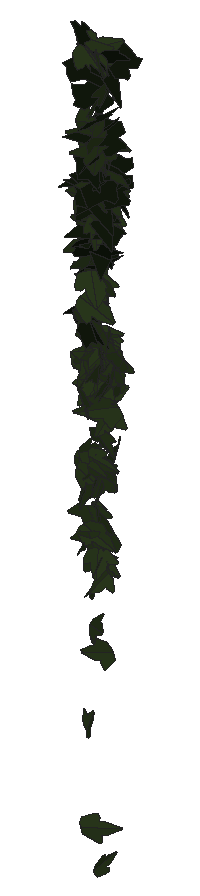
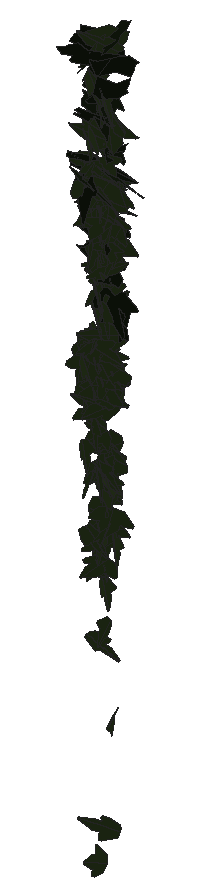
# SketchUp Ruby script. Lengths in inches.
U = 1.inch
M = Sketchup.active_model
def pt(a) = Geom::Point3d.new(a.map { |v| v * U })
def face(e, loops, mat)
  f = e.add_face(loops[0].map { |a| pt(a) })
  loops[1..].each { |l| e.add_face(l.map { |a| pt(a) }).erase! }
  f.material = f.back_material = mat if mat
  f
end
# faces: each face lists its corners as indices into pts; further lists are holes
def faces(e, pts, list, mat = nil) = list.each { |f| face(e, (f[0].is_a?(Array) ? f : [f]).map { |l| l.map { |i| pts[i] } }, mat) }
# xy, xz, yz: faces in a plane at the given z, y or x. An outline is a flat list of corners, or four numbers for a rectangle; further outlines are holes
def ring(l) = l.size == 4 ? [[l[0], l[1]], [l[2], l[1]], [l[2], l[3]], [l[0], l[3]]] : l.each_slice(2).to_a
def flat(e, list, mat, &to3) = list.each { |f| face(e, (f[0].is_a?(Array) ? f : [f]).map { |l| ring(l).map { |u, v| to3.(u, v) } }, mat) }
def xy(e, z, list, mat = nil) = flat(e, list, mat) { |x, y| [x, y, z] }
def xz(e, y, list, mat = nil) = flat(e, list, mat) { |x, z| [x, y, z] }
def yz(e, x, list, mat = nil) = flat(e, list, mat) { |y, z| [x, y, z] }
def lines(e, pts, list) = list.each { |a, b| e.add_line(pt(pts[a]), pt(pts[b])) }
# prism: a flat outline (further loops are holes) pulled along v
def prism(e, loops, v, mat = nil)
  f = face(e, loops, mat); d = Geom::Vector3d.new(v.map { |x| x * U })
  f.pushpull(f.normal.samedirection?(d) ? d.length : -d.length)
end
def box(e, o, s, mat = nil) = prism(e, [[o, [o[0] + s[0], o[1], o[2]], [o[0] + s[0], o[1] + s[1], o[2]], [o[0], o[1] + s[1], o[2]]]], [0, 0, s[2]], mat)
def at(x, y, z, deg = 0) = Geom::Transformation.translation(pt([x, y, z])) * Geom::Transformation.rotation(ORIGIN, Z_AXIS, deg.degrees)
def axes(o, x, y, z) = Geom::Transformation.new([*x, 0, *y, 0, *z, 0, *pt(o).to_a, 1])
def part(name) = M.definitions.add(name)
# library, detail: a bought-in or finely detailed component or shape, given as its bounding box
def library(name, o, s) = part(name).tap { |d| box(d.entities, o, s) }
def detail(e, o, s) = box(e.add_group.entities, o, s)
def put(e, d, t, mat = nil) = e.add_instance(d, t).tap { |i| i.material = mat if mat }
def group(e, t, mat = nil) = e.add_group.tap { |g| g.transformation = t; g.material = mat if mat }.entities
root = M.entities
M.materials.add("1026 AP 7946 SUNNY SIDE UP").color = [254, 231, 186]
M.materials.add("efeu1").color = [18, 25, 13]
M.materials.add("efeu2").color = [43, 57, 29]
c1 = part("ivyleaf_10")
p = [[0,0.5,-0.03],[-0.0625,2.02,-0.43],[-0.19,2.01,-0.46],[-0.54,1.05,-0.29],[-0.52,0.625,-0.18],[-0.83,0.76,-0.28],
  [-1.16,0.64,-0.33],[-1.15,0.33,-0.24],[-0.77,-0.39,0.02],[-0.3,-0.51,0.16],[0.04,-0.48,0.23],[-0.02,2.01,-0.4375],
  [-0.06,2.01,-0.43],[0.04,-0.49,0.23],[0.67,-0.49,0.14],[1.38,0.36,-0.2],[1.375,0.51,-0.24],[0.81,0.65,-0.19],
  [0.62,0.59,-0.15],[0.6,1.09,-0.28],[0.5,1.23,-0.31]]
faces(c1.entities,p,[[0,1,2,3,4,5,6,7,8,9,10],[11,12,0,13,14,15,16,17,18,19,20]],"efeu2")
c2 = part("ivyleaf_9")
p = [[1.54,2.16,1.25],[1.36,2.04,1.19],[-0.21,0.99,0.68],[-0.71,1.11,0.82],[-0.85,0.86,0.67],[-0.8,0.17,0.21],
  [-0.9,-0.01,0.1],[-0.67,-0.16,-0.02],[-0.08,-0.08,-0.05],[-0.03,-0.6,-0.4],[0.65,-0.88,-0.66],[0.83,-0.6,-0.49],
  [1.29,-0.42,-0.43],[1.8125,-0.07,-0.26],[1.21,0.44,0.15]]
faces(c2.entities,p,[[0,1,2,3,4,5,6,7,8,9,10,11,12,13,14]],"efeu1")
put(root,c1,axes([98.8,213.06,258.14],[-0.01236,0.17626,-0.01871],[0.00185,-0.01974,-0.18914],[-0.30108,-0.00736,-0.00039]),"1026 AP 7946 SUNNY SIDE UP")
put(root,c1,axes([98.79,212.91,264.06],[-0.33972,0.04678,-0.08865],[0.10232,-0.08801,-0.21744],[-0.1156,-0.21537,0.06807]),"1026 AP 7946 SUNNY SIDE UP")
put(root,c1,axes([98.8,212.71,264.67],[0.31073,-0.13559,0.04289],[0.03828,-0.03961,-0.24366],[0.23782,0.18354,-0.01682]),"1026 AP 7946 SUNNY SIDE UP")
put(root,c2,axes([98.93,212.62,262.46],[0.05883,0.21135,-0.04868],[-0.00859,-0.04804,-0.22994],[-0.3679,0.03492,-0.00242]),"1026 AP 7946 SUNNY SIDE UP")
put(root,c1,axes([98.84,212.95,264.04],[-0.21605,0.18995,-0.03933],[-0.00162,-0.04882,-0.23994],[-0.30498,-0.1343,0.02913]),"1026 AP 7946 SUNNY SIDE UP")
put(root,c1,axes([98.87,212.85,261.1],[-0.05485,-0.17256,0.13795],[0.0276,-0.13835,-0.17846],[0.34328,-0.01645,0.03639]),"1026 AP 7946 SUNNY SIDE UP")
put(root,c1,axes([98.9,212.66,257.76],[0.06366,-0.19471,-0.10885],[-0.02274,0.10373,-0.20418],[0.34677,0.04255,0.00659]),"1026 AP 7946 SUNNY SIDE UP")
put(root,c1,axes([99,212.97,263.11],[-0.02811,-0.03849,-0.21853],[-0.22871,-0.15321,0.0406],[-0.26728,0.13514,-0.01176]),"1026 AP 7946 SUNNY SIDE UP")
put(root,c2,axes([98.66,212.87,267.79],[0.19964,-0.22569,-0.00204],[-0.00861,-0.00228,-0.26671],[0.35477,0.12695,-0.00532]),"1026 AP 7946 SUNNY SIDE UP")
put(root,c1,axes([98.67,212.93,261.24],[0.27425,0.06827,0.12923],[0.18057,0.04964,-0.19263],[-0.1326,0.20879,0.00496]),"1026 AP 7946 SUNNY SIDE UP")
put(root,c1,axes([98.85,212.74,263.6],[-0.26261,-0.15515,-0.05485],[0.08716,0.0168,-0.23335],[0.24228,-0.17422,0.0245]),"1026 AP 7946 SUNNY SIDE UP")
put(root,c1,axes([98.84,212.6,260.65],[-0.18983,0.14942,-0.04664],[0.03068,-0.04323,-0.20005],[-0.26338,-0.11273,0.01032]),"1026 AP 7946 SUNNY SIDE UP")
put(root,c1,axes([98.92,212.74,262.22],[-0.06474,-0.10987,-0.20639],[-0.09921,-0.18953,0.1197],[-0.34442,0.07525,0.00431]),"1026 AP 7946 SUNNY SIDE UP")
put(root,c1,axes([98.97,212.66,261.11],[0.12421,-0.01266,0.17228],[-0.17251,0.13388,0.06256],[-0.21326,-0.11567,0.04974]),"1026 AP 7946 SUNNY SIDE UP")
put(root,c1,axes([98.93,212.56,258.82],[0.02989,-0.11046,-0.19738],[-0.01645,0.19101,-0.11378],[0.34651,0.0186,0.01163]),"1026 AP 7946 SUNNY SIDE UP")
put(root,c1,axes([98.68,212.83,265.98],[0.10054,-0.08905,-0.20527],[0.20973,-0.14551,0.11187],[-0.289,-0.13658,0.00977]),"1026 AP 7946 SUNNY SIDE UP")
put(root,c2,axes([99.1,212.83,265.08],[-0.33878,0.10238,-0.01465],[-0.02343,-0.05867,-0.23267],[-0.17408,-0.19134,0.05982]),"1026 AP 7946 SUNNY SIDE UP")
put(root,c1,axes([99.08,212.99,261.58],[-0.13659,-0.07862,0.1759],[-0.17591,-0.12932,-0.12163],[0.25619,-0.13071,0.01026]),"1026 AP 7946 SUNNY SIDE UP")
put(root,c1,axes([99.03,212.79,264.04],[-0.34364,-0.04308,0.08102],[-0.10256,-0.0667,-0.22406],[0.09725,-0.22257,0.05]),"1026 AP 7946 SUNNY SIDE UP")
put(root,c1,axes([98.92,212.75,258.28],[-0.3045,-0.09119,-0.03618],[0.06281,-0.00397,-0.21954],[0.13991,-0.19668,0.01981]),"1026 AP 7946 SUNNY SIDE UP")
put(root,c1,axes([98.88,212.97,263.19],[0.08219,0.19373,-0.01329],[0.0004,-0.01545,-0.21395],[-0.32984,0.04825,-0.00357]),"1026 AP 7946 SUNNY SIDE UP")
put(root,c1,axes([99.05,212.86,263.56],[-0.28814,-0.038,0.081],[-0.11314,-0.04632,-0.18443],[0.08986,-0.18019,0.02754]),"1026 AP 7946 SUNNY SIDE UP")
put(root,c1,axes([99.01,212.73,265.84],[-0.36449,-0.08428,0.03528],[-0.03523,-0.03958,-0.24555],[0.15023,-0.21377,0.02801]),"1026 AP 7946 SUNNY SIDE UP")
put(root,c1,axes([98.97,212.86,266.5],[0.11272,-0.23993,-0.03251],[-0.01248,0.02914,-0.2578],[0.38004,0.07212,0.00118]),"1026 AP 7946 SUNNY SIDE UP")
put(root,c1,axes([98.76,212.99,264.07],[0.27442,0.10855,0.12306],[0.15786,0.06358,-0.21136],[-0.1978,0.20134,0.00204]),"1026 AP 7946 SUNNY SIDE UP")
put(root,c1,axes([98.98,212.66,263.41],[-0.08145,-0.22528,-0.02578],[0.00269,0.02397,-0.23797],[0.35619,-0.0517,-0.0041]),"1026 AP 7946 SUNNY SIDE UP")
put(root,c1,axes([98.89,212.83,261.24],[-0.3321,-0.02047,-0.06843],[0.11093,-0.01693,-0.20945],[0.024,-0.20503,0.02121]),"1026 AP 7946 SUNNY SIDE UP")
put(root,c1,axes([98.93,212.7,261.35],[-0.01118,0.151,0.13423],[-0.03822,0.12207,-0.15947],[-0.32883,-0.01932,0.01397]),"1026 AP 7946 SUNNY SIDE UP")
put(root,c1,axes([98.96,212.98,265.25],[0.22882,0.15799,-0.11597],[-0.09814,-0.09629,-0.22114],[-0.28968,0.15742,-0.01668]),"1026 AP 7946 SUNNY SIDE UP")
put(root,c1,axes([98.85,212.87,260.5],[0.07504,0.06221,0.2228],[0.06395,0.21469,-0.07173],[-0.34748,0.05295,0.03491]),"1026 AP 7946 SUNNY SIDE UP")
put(root,c1,axes([98.99,212.67,264.82],[-0.21121,-0.17964,0.03041],[0.02042,-0.04524,-0.2315],[0.30871,-0.11991,0.03611]),"1026 AP 7946 SUNNY SIDE UP")
put(root,c2,axes([98.81,212.74,267.25],[-0.04661,-0.09341,-0.21523],[0.08823,0.19296,-0.10152],[0.3639,-0.05875,-0.00295]),"1026 AP 7946 SUNNY SIDE UP")
put(root,c2,axes([98.95,212.77,266.46],[-0.196,-0.06937,0.20857],[0.25278,0.12842,0.14457],[-0.24568,0.18747,-0.01765]),"1026 AP 7946 SUNNY SIDE UP")
put(root,c2,axes([98.7,212.75,262.11],[0.06794,-0.02366,-0.22592],[0.35914,-0.00999,0.04408],[-0.02425,-0.21426,0.01986]),"1026 AP 7946 SUNNY SIDE UP")
put(root,c1,axes([98.95,212.73,258.96],[0.07661,-0.16665,0.12313],[0.0426,-0.11752,-0.17946],[0.32052,0.05546,-0.00558]),"1026 AP 7946 SUNNY SIDE UP")
put(root,c1,axes([99.09,212.75,261.33],[-0.27198,-0.07417,0.11602],[-0.1085,-0.1069,-0.17939],[0.1963,-0.16186,0.0616]),"1026 AP 7946 SUNNY SIDE UP")
put(root,c1,axes([98.99,212.86,262.34],[0.21398,-0.16783,-0.08574],[-0.02862,0.08938,-0.21834],[0.29251,0.13152,0.04136]),"1026 AP 7946 SUNNY SIDE UP")
put(root,c1,axes([98.98,213,259.14],[0.16048,-0.16931,-0.0622],[0.00085,0.06864,-0.20015],[0.28213,0.0961,0.03598]),"1026 AP 7946 SUNNY SIDE UP")
put(root,c1,axes([98.97,212.79,258.74],[0.04094,-0.154,0.15626],[0.04094,-0.15032,-0.16178],[0.33838,0.03682,0.00067]),"1026 AP 7946 SUNNY SIDE UP")
put(root,c1,axes([99,212.85,263.24],[0.04539,-0.21692,0.074],[0.01609,-0.07235,-0.22586],[0.35955,0.03062,0.00076]),"1026 AP 7946 SUNNY SIDE UP")
put(root,c1,axes([99.1875,212.8,259.12],[-0.19335,0.00844,0.15833],[-0.2507,-0.01901,-0.12096],[0.01688,-0.18561,0.01696]),"1026 AP 7946 SUNNY SIDE UP")
put(root,c1,axes([99.0625,213.01,261.04],[-0.33693,0.00923,0.04265],[-0.06616,-0.02118,-0.21985],[-0.00787,-0.2172,0.02197]),"1026 AP 7946 SUNNY SIDE UP")
put(root,c1,axes([99.04,212.77,261.03],[0.09464,-0.18322,-0.11419],[-0.04166,0.10679,-0.19792],[0.33327,0.06538,0.00768]),"1026 AP 7946 SUNNY SIDE UP")
put(root,c1,axes([98.94,213,260.76],[-0.26939,-0.11976,-0.05723],[0.11204,-0.00854,-0.21005],[0.17421,-0.17969,0.04661]),"1026 AP 7946 SUNNY SIDE UP")
put(root,c1,axes([98.9375,212.91,264.75],[-0.35936,-0.02762,-0.07319],[0.11626,-0.02769,-0.2346],[0.02822,-0.23768,0.0344]),"1026 AP 7946 SUNNY SIDE UP")
put(root,c1,axes([98.97,212.53,259.55],[0.01289,-0.00165,0.19759],[-0.02705,0.18404,0.00503],[-0.31218,-0.01601,0.00772]),"1026 AP 7946 SUNNY SIDE UP")
put(root,c1,axes([98.96,212.47,259.2],[-0.00309,0.15177,0.14418],[-0.01325,0.13255,-0.16057],[-0.34197,-0.00651,0.00492]),"1026 AP 7946 SUNNY SIDE UP")
put(root,c1,axes([99.03,212.85,261.39],[-0.03764,-0.19899,0.10063],[0.00461,-0.09965,-0.2066],[0.34931,-0.02013,0.01357]),"1026 AP 7946 SUNNY SIDE UP")
put(root,c1,axes([99.02,212.65,264.69],[-0.32219,0.12867,-0.00292],[-0.01136,-0.01818,-0.24858],[-0.20208,-0.20413,0.01863]),"1026 AP 7946 SUNNY SIDE UP")
put(root,c1,axes([98.99,212.89,264.45],[0.35929,0.06861,-0.02862],[-0.04944,0.00696,-0.24521],[-0.10562,0.23012,0.01742]),"1026 AP 7946 SUNNY SIDE UP")
put(root,c2,axes([98.85,212.68,263.05],[0.11021,0.19585,-0.04087],[0.00814,0.04129,0.22129],[0.33948,-0.06457,0.00796]),"1026 AP 7946 SUNNY SIDE UP")
put(root,c2,axes([99.09,212.49,265.41],[0.05671,0.14674,0.1823],[0.00922,0.16966,-0.15708],[-0.37902,0.02608,0.02346]),"1026 AP 7946 SUNNY SIDE UP")
put(root,c1,axes([98.79,212.81,261.86],[-0.03513,-0.02996,-0.23643],[0.32677,0.09852,-0.03354],[0.15961,-0.2083,0.01663]),"1026 AP 7946 SUNNY SIDE UP")
put(root,c1,axes([99.1,212.91,262.78],[0.10117,-0.12,-0.17445],[-0.07943,0.15543,-0.14006],[0.33202,0.07375,0.01965]),"1026 AP 7946 SUNNY SIDE UP")
put(root,c1,axes([99.0625,212.74,256.86],[0.03099,-0.19862,-0.05182],[-0.01271,0.04861,-0.20532],[0.3215,0.02107,-0.00312]),"1026 AP 7946 SUNNY SIDE UP")
put(root,c1,axes([99.08,212.74,260.84],[0.31617,0.03751,-0.09145],[-0.12859,-0.04317,-0.20937],[-0.08076,0.21561,-0.02466]),"1026 AP 7946 SUNNY SIDE UP")
put(root,c1,axes([99.07,212.8125,266.07],[0.09531,-0.22255,-0.10344],[-0.01312,0.10021,-0.2364],[0.38286,0.05883,0.01765]),"1026 AP 7946 SUNNY SIDE UP")
put(root,c1,axes([99.05,213,262.31],[0.13901,-0.20792,-0.0236],[0.00633,0.02528,-0.23219],[0.32866,0.08746,0.01445]),"1026 AP 7946 SUNNY SIDE UP")
put(root,c1,axes([99.08,212.46,254.12],[0.03363,0.01409,-0.20958],[-0.01478,0.20449,0.01476],[0.32044,0.00795,0.02267]),"1026 AP 7946 SUNNY SIDE UP")
put(root,c2,axes([99.08,212.52,263.9],[0.09776,0.20391,0.03277],[0.02273,0.02525,-0.2264],[-0.34865,0.05882,-0.00557]),"1026 AP 7946 SUNNY SIDE UP")
put(root,c1,axes([99.08,212.66,256.02],[-0.00172,0.11735,0.16115],[-0.093,0.14247,-0.11854],[-0.30824,-0.04364,0.03487]),"1026 AP 7946 SUNNY SIDE UP")
put(root,c1,axes([99.15,212.73,258.96],[-0.29891,-0.04066,0.05448],[-0.07706,-0.03069,-0.19284],[0.08028,-0.18085,0.01774]),"1026 AP 7946 SUNNY SIDE UP")
put(root,c1,axes([99.14,212.85,264.05],[-0.32664,-0.08774,0.03731],[-0.04448,-0.02907,-0.22621],[0.15472,-0.19358,0.01374]),"1026 AP 7946 SUNNY SIDE UP")
put(root,c1,axes([98.83,212.65,259.3],[-0.04966,-0.00705,-0.22537],[0.28476,-0.1249,-0.02352],[-0.19317,-0.18231,0.02326]),"1026 AP 7946 SUNNY SIDE UP")
put(root,c1,axes([99.18,212.9,264.58],[-0.33432,0.08394,0.05804],[-0.13046,-0.05403,-0.21441],[-0.10683,-0.1967,0.08021]),"1026 AP 7946 SUNNY SIDE UP")
put(root,c2,axes([98.95,212.71,265.32],[0.07984,-0.20966,-0.10106],[-0.04598,0.08782,-0.2287],[0.3857,0.05387,-0.00635]),"1026 AP 7946 SUNNY SIDE UP")
put(root,c2,axes([99.33,212.91,264.75],[-0.14477,0.19178,0.11984],[-0.15691,0.07634,-0.21257],[-0.31489,-0.12622,0.05083]),"1026 AP 7946 SUNNY SIDE UP")
put(root,c1,axes([98.83,212.87,267.48],[0.21002,-0.00539,-0.1988],[0.30242,0.06642,0.12598],[0.089,-0.21296,0.04106]),"1026 AP 7946 SUNNY SIDE UP")
put(root,c1,axes([99.08,212.56,257.91],[-0.24183,-0.09933,-0.03393],[0.05717,0.00464,-0.18514],[0.16681,-0.14559,0.01427]),"1026 AP 7946 SUNNY SIDE UP")
put(root,c1,axes([98.93,212.93,264.11],[-0.1128,0.07636,0.2051],[0.25015,-0.12174,0.10553],[0.24268,0.16098,-0.01344]),"1026 AP 7946 SUNNY SIDE UP")
put(root,c1,axes([99.1,213,260.11],[0.18806,-0.15399,-0.0904],[-0.02291,0.09595,-0.1953],[0.27707,0.11246,0.04521]),"1026 AP 7946 SUNNY SIDE UP")
put(root,c1,axes([99.15,212.95,261.62],[0.19442,0.08341,-0.12457],[-0.14188,-0.08373,-0.15209],[-0.19917,0.14107,-0.01326]),"1026 AP 7946 SUNNY SIDE UP")
put(root,c1,axes([99.11,212.99,263.52],[0.00137,-0.13864,-0.16483],[0.01874,0.15196,-0.14606],[0.34893,-0.00762,0.00849]),"1026 AP 7946 SUNNY SIDE UP")
put(root,c1,axes([99.11,212.93,265.78],[0.04186,-0.22392,0.13874],[0.01919,-0.13544,-0.23308],[0.41146,0.0291,-0.00325]),"1026 AP 7946 SUNNY SIDE UP")
put(root,c1,axes([98.98,212.59,267.6],[0.17055,0.2057,0.12081],[0.06365,0.10968,-0.23851],[-0.36592,0.11496,0.01482]),"1026 AP 7946 SUNNY SIDE UP")
put(root,c2,axes([99.02,212.52,262.15],[0.1361,-0.10344,-0.18369],[-0.12905,0.15373,-0.13618],[0.31255,0.10852,0.02376]),"1026 AP 7946 SUNNY SIDE UP")
put(root,c1,axes([99.29,212.8125,264.17],[0.22514,-0.0188,-0.17721],[-0.28203,-0.00441,-0.14225],[0.01411,0.21187,-0.01571]),"1026 AP 7946 SUNNY SIDE UP")
put(root,c1,axes([99.15,212.85,264.2],[0.14156,-0.19938,-0.10704],[-0.03207,0.103,-0.22367],[0.35125,0.08976,0.02271]),"1026 AP 7946 SUNNY SIDE UP")
put(root,c1,axes([99.17,213,260.84],[-0.2195,-0.15074,0.07019],[-0.01008,-0.08522,-0.20568],[0.26048,-0.13033,0.05119]),"1026 AP 7946 SUNNY SIDE UP")
put(root,c1,axes([99.07,212.84,259.15],[0.11634,-0.14124,0.11761],[0.07707,-0.1021,-0.16946],[0.29579,0.08215,-0.0021]),"1026 AP 7946 SUNNY SIDE UP")
put(root,c2,axes([99.14,212.75,267.52],[0.19915,0.17491,-0.05335],[-0.03648,-0.04829,-0.22595],[-0.30765,0.11894,-0.00774]),"1026 AP 7946 SUNNY SIDE UP")
put(root,c1,axes([99.17,212.94,266.83],[0.01867,-0.25189,0.0189],[0.00032,-0.01978,-0.2599],[0.39729,0.01186,-0.00068]),"1026 AP 7946 SUNNY SIDE UP")
put(root,c1,axes([99.32,212.85,257.84],[-0.20186,0.05617,0.15104],[-0.24136,-0.00699,-0.13604],[-0.04962,-0.19451,0.04727]),"1026 AP 7946 SUNNY SIDE UP")
put(root,c1,axes([99.1,212.87,260.82],[0.0351,0.19481,0.12954],[-0.01887,0.12602,-0.19997],[-0.36315,0.01228,0.02291]),"1026 AP 7946 SUNNY SIDE UP")
put(root,c1,axes([98.93,212.98,260.47],[0.20689,-0.0157,-0.17712],[0.25298,0.08929,0.11903],[0.0981,-0.19715,0.06662]),"1026 AP 7946 SUNNY SIDE UP")
put(root,c1,axes([99.17,212.74,262.98],[-0.2942,0.10457,0.01589],[-0.03483,-0.00801,-0.216],[-0.17556,-0.17365,0.01622]),"1026 AP 7946 SUNNY SIDE UP")
put(root,c1,axes([99.24,212.86,261.58],[-0.22177,-0.10551,0.14218],[-0.06936,-0.1509,-0.16546],[0.26499,-0.1278,0.07568]),"1026 AP 7946 SUNNY SIDE UP")
put(root,c1,axes([99.17,212.68,257.375],[0.10805,-0.18638,-0.05835],[-0.01825,0.05491,-0.20416],[0.30527,0.06925,0.00845]),"1026 AP 7946 SUNNY SIDE UP")
put(root,c1,axes([99.12,212.8,259.32],[0.05723,-0.17025,-0.12829],[0.06975,0.12879,-0.1686],[0.32334,0.00235,0.05908]),"1026 AP 7946 SUNNY SIDE UP")
put(root,c2,axes([99.08,212.55,263.67],[0.27683,0.13526,0.00451],[0.01814,-0.00905,-0.22647],[-0.22892,0.16284,-0.01249]),"1026 AP 7946 SUNNY SIDE UP")
put(root,c1,axes([99.24,212.65,258.31],[-0.25889,0.12447,0.07848],[-0.11264,0.0299,-0.21163],[-0.19925,-0.17863,0.01768]),"1026 AP 7946 SUNNY SIDE UP")
put(root,c1,axes([99.11,213.03,261.66],[0.04764,0.17422,-0.01266],[-0.00077,-0.01421,-0.18911],[-0.29671,0.02801,-0.00154]),"1026 AP 7946 SUNNY SIDE UP")
put(root,c2,axes([99.07,212.84,263.69],[-0.06207,-0.21468,0.01843],[-0.0019,-0.02011,-0.23341],[0.36601,-0.03651,0.00191]),"1026 AP 7946 SUNNY SIDE UP")
put(root,c1,axes([99.2,212.87,260.8125],[0.09302,-0.20818,-0.04198],[-0.02596,0.03643,-0.22266],[0.33218,0.06114,-0.00565]),"1026 AP 7946 SUNNY SIDE UP")
put(root,c1,axes([99.21,212.59,265.67],[-0.27453,-0.17355,0.01655],[0.00269,-0.02562,-0.25354],[0.29612,-0.16066,0.01764]),"1026 AP 7946 SUNNY SIDE UP")
put(root,c2,axes([99.24,212.68,265.02],[-0.36271,-0.06072,-0.05288],[0.08635,-0.0092,-0.2447],[0.08994,-0.23606,0.02167]),"1026 AP 7946 SUNNY SIDE UP")
put(root,c1,axes([99.11,212.99,265.18],[-0.0441,0.19386,-0.05742],[0.01028,-0.05585,-0.21017],[-0.34246,-0.02664,0.00109]),"1026 AP 7946 SUNNY SIDE UP")
put(root,c2,axes([99.44,212.8,265.93],[-0.32675,0.03999,0.11808],[-0.19442,-0.02279,-0.20642],[-0.03917,-0.22041,0.03956]),"1026 AP 7946 SUNNY SIDE UP")
put(root,c1,axes([99.19,212.64,261.29],[0.00878,-0.21224,-0.07342],[0.00524,0.07015,-0.21825],[0.35139,0.00426,0.00509]),"1026 AP 7946 SUNNY SIDE UP")
put(root,c1,axes([99.22,212.62,264.3],[-0.12194,-0.21632,0.04745],[-0.00386,-0.04884,-0.2443],[0.3758,-0.07069,0.01289]),"1026 AP 7946 SUNNY SIDE UP")
put(root,c1,axes([99.05,212.79,257.31],[-0.1888,-0.10087,-0.13537],[0.19775,0.04906,-0.15759],[0.16844,-0.17066,0.03328]),"1026 AP 7946 SUNNY SIDE UP")
put(root,c1,axes([99.27,212.88,265.41],[0.10998,-0.0492,0.20631],[-0.19701,0.15606,0.08632],[-0.27548,-0.13125,0.02063]),"1026 AP 7946 SUNNY SIDE UP")
put(root,c1,axes([99.14,212.74,267.49],[-0.07145,0.21973,0.01172],[-0.017,0.00631,-0.23924],[-0.37286,-0.04239,0.00866]),"1026 AP 7946 SUNNY SIDE UP")
put(root,c2,axes([99.44,213.09,267.22],[-0.10948,0.04562,0.21248],[-0.34467,-0.01103,-0.06828],[-0.00574,-0.20783,0.04721]),"1026 AP 7946 SUNNY SIDE UP")
put(root,c1,axes([99.39,212.69,260.51],[0.15086,0.03476,-0.2207],[-0.3257,-0.056,-0.10516],[-0.10292,0.22815,0.00926]),"1026 AP 7946 SUNNY SIDE UP")
put(root,c1,axes([99.24,212.69,257.625],[0.16046,-0.05724,-0.19046],[-0.06891,0.19641,-0.08657],[0.29591,0.07678,0.08312]),"1026 AP 7946 SUNNY SIDE UP")
put(root,c1,axes([99.15,213,264.17],[0.11905,0.17681,-0.08025],[-0.03486,-0.0749,-0.20451],[-0.32569,0.07265,-0.00744]),"1026 AP 7946 SUNNY SIDE UP")
put(root,c2,axes([99.29,212.46,266.34],[0.04439,0.20908,0.10009],[-0.03607,0.0932,-0.22199],[-0.38524,0.01537,0.03232]),"1026 AP 7946 SUNNY SIDE UP")
put(root,c1,axes([99.37,212.625,255.64],[0.15392,-0.06381,-0.17446],[-0.24989,0.06094,-0.11819],[0.13501,0.18554,-0.01985]),"1026 AP 7946 SUNNY SIDE UP")
put(root,c1,axes([99.1,212.58,263.07],[0.24246,0.18021,0.00778],[0.0311,-0.00826,-0.24541],[-0.30445,0.14268,-0.01887]),"1026 AP 7946 SUNNY SIDE UP")
put(root,c1,axes([99.14,212.77,261.63],[-0.0509,0.18008,-0.06118],[0.01203,-0.05913,-0.19625],[-0.32172,-0.03071,0.00234]),"1026 AP 7946 SUNNY SIDE UP")
put(root,c1,axes([99.09,212.8,259.85],[-0.23144,0.06158,-0.10767],[0.14369,-0.05769,-0.16019],[-0.14106,-0.1598,0.01348]),"1026 AP 7946 SUNNY SIDE UP")
put(root,c1,axes([99.22,212.93,261.1],[-0.10847,-0.20623,-0.0183],[0.03454,0.01009,-0.22323],[0.32348,-0.07023,0.0177]),"1026 AP 7946 SUNNY SIDE UP")
put(root,c1,axes([99.0625,212.51,262.6],[0.09492,0.18033,0.17692],[0.10714,0.15691,-0.19466],[-0.37546,0.09036,-0.01082]),"1026 AP 7946 SUNNY SIDE UP")
put(root,c2,axes([99.33,212.59,266.1],[-0.02658,0.21254,0.06209],[-0.0163,0.05465,-0.22733],[-0.37243,-0.01756,0.00552]),"1026 AP 7946 SUNNY SIDE UP")
put(root,c1,axes([99.21,212.95,259.03],[-0.08912,0.16635,0.07154],[-0.04671,0.05905,-0.18573],[-0.29934,-0.05874,0.00768]),"1026 AP 7946 SUNNY SIDE UP")
put(root,c2,axes([99.48,212.95,265.16],[-0.31539,0.12292,0.06508],[-0.12651,-0.01477,-0.23625],[-0.17608,-0.20956,0.05317]),"1026 AP 7946 SUNNY SIDE UP")
put(root,c1,axes([99.41,212.77,261.61],[-0.21071,0.04576,0.15521],[-0.25019,0.00653,-0.13777],[-0.05925,-0.19029,0.02979]),"1026 AP 7946 SUNNY SIDE UP")
put(root,c1,axes([99.24,212.83,261.79],[0.12676,-0.20304,-0.06335],[-0.02039,0.05971,-0.22449],[0.33244,0.08108,0.01039]),"1026 AP 7946 SUNNY SIDE UP")
put(root,c1,axes([99.2,213.02,261.24],[-0.33934,-0.02288,-0.03456],[0.05577,-0.01929,-0.22246],[0.03075,-0.21753,0.02207]),"1026 AP 7946 SUNNY SIDE UP")
put(root,c2,axes([99.41,212.71,264.21],[-0.32561,-0.05933,0.10728],[-0.14475,-0.0621,-0.21332],[0.13629,-0.20768,0.02975]),"1026 AP 7946 SUNNY SIDE UP")
put(root,c1,axes([99.26,213.01,261.26],[0.01618,-0.21841,0.01872],[-0.00499,-0.01958,-0.22533],[0.34475,0.00997,-0.00414]),"1026 AP 7946 SUNNY SIDE UP")
put(root,c2,axes([99.3,212.96,264.74],[0.21798,-0.01272,-0.20364],[-0.30347,0.04523,-0.14222],[0.06958,0.2371,0.01765]),"1026 AP 7946 SUNNY SIDE UP")
put(root,c1,axes([99.27,212.94,264.71],[-0.21013,-0.19667,0.04267],[0.01679,-0.05793,-0.24167],[0.31594,-0.12772,0.04123]),"1026 AP 7946 SUNNY SIDE UP")
put(root,c1,axes([99.29,212.54,262.07],[0.26423,-0.11851,-0.10664],[-0.08332,0.09898,-0.20611],[0.23223,0.17035,0.04738]),"1026 AP 7946 SUNNY SIDE UP")
put(root,c2,axes([99.07,212.9375,267.26],[0.09878,-0.24737,0.00449],[0.00283,-0.00549,-0.26296],[0.38906,0.06285,0.00078]),"1026 AP 7946 SUNNY SIDE UP")
put(root,c2,axes([99.07,212.65,264.71],[0.01323,-0.21735,-0.03161],[0.08311,0.02776,-0.22633],[0.36232,0.00157,0.05307]),"1026 AP 7946 SUNNY SIDE UP")
put(root,c1,axes([99.45,212.92,261.42],[-0.13938,0.02744,0.17312],[-0.27496,0.01226,-0.0903],[-0.03984,-0.18062,0.01758]),"1026 AP 7946 SUNNY SIDE UP")
put(root,c1,axes([99.27,212.75,260.97],[0.01034,-0.19409,-0.11414],[0.00853,0.10985,-0.19926],[0.35045,0.00305,0.00822]),"1026 AP 7946 SUNNY SIDE UP")
put(root,c1,axes([99.28,212.85,260.24],[0.20122,0.12789,-0.08941],[-0.12489,-0.04721,-0.18615],[-0.229,0.13812,0.02296]),"1026 AP 7946 SUNNY SIDE UP")
put(root,c1,axes([99.29,212.85,260.75],[-0.09062,-0.20903,0.04487],[-0.00301,-0.04584,-0.2234],[0.33611,-0.05677,0.0101]),"1026 AP 7946 SUNNY SIDE UP")
put(root,c1,axes([99.22,212.5,266],[-0.04726,-0.10845,-0.23167],[0.09208,0.20802,-0.11697],[0.39824,-0.06097,-0.00044]),"1026 AP 7946 SUNNY SIDE UP")
put(root,c1,axes([99.06,212.5625,258.01],[0.1803,0.07556,0.16262],[0.19713,0.09548,-0.14072],[-0.19114,0.16975,0.00827]),"1026 AP 7946 SUNNY SIDE UP")
put(root,c1,axes([99.24,212.57,264.27],[0.14834,0.2161,-0.03183],[-0.06159,-0.02023,-0.2483],[-0.36583,0.09103,0.02889]),"1026 AP 7946 SUNNY SIDE UP")
put(root,c1,axes([99.22,212.6,257.55],[0.17757,0.16891,-0.03874],[-0.03051,-0.03402,-0.21316],[-0.29246,0.1061,-0.00129]),"1026 AP 7946 SUNNY SIDE UP")
put(root,c1,axes([99.29,212.57,258.875],[0.10998,-0.19362,-0.06159],[-0.02247,0.05721,-0.21166],[0.31733,0.07115,0.00636]),"1026 AP 7946 SUNNY SIDE UP")
put(root,c1,axes([99.28,212.82,265.09],[-0.37717,0.04666,-0.01404],[0.01118,-0.03549,-0.24958],[-0.07573,-0.23763,0.03304]),"1026 AP 7946 SUNNY SIDE UP")
put(root,c1,axes([99.29,212.71,257.07],[0.09031,0.08641,-0.15696],[-0.1002,-0.13596,-0.10979],[-0.27272,0.07857,-0.01164]),"1026 AP 7946 SUNNY SIDE UP")
put(root,c1,axes([99.04,212.625,259.45],[-0.09339,-0.02176,-0.18578],[0.2895,-0.04568,-0.05247],[-0.06361,-0.17594,0.03394]),"1026 AP 7946 SUNNY SIDE UP")
put(root,c1,axes([99.02,213,265.75],[-0.05215,-0.00853,-0.21867],[0.30565,-0.09871,-0.02597],[-0.16395,-0.18132,0.02114]),"1026 AP 7946 SUNNY SIDE UP")
put(root,c1,axes([99.03,212.59,252.02],[0.06211,-0.00645,-0.20622],[0.30882,0.04099,0.03881],[0.06134,-0.19984,0.01339]),"1026 AP 7946 SUNNY SIDE UP")
put(root,c1,axes([99.3,213,259.58],[0.03306,-0.20273,-0.04952],[0.00275,0.04733,-0.20959],[0.32719,0.02008,0.00677]),"1026 AP 7946 SUNNY SIDE UP")
put(root,c2,axes([99.13,212.67,264.41],[-0.03214,-0.21256,-0.04203],[0.07727,0.03187,-0.22357],[0.35786,-0.02597,0.0445]),"1026 AP 7946 SUNNY SIDE UP")
put(root,c2,axes([99.6,212.75,264.93],[-0.27167,0.05039,0.18371],[-0.27963,0.02204,-0.18409],[-0.08034,-0.24711,0.01953]),"1026 AP 7946 SUNNY SIDE UP")
put(root,c1,axes([99.26,212.59,251.28],[0.04855,-0.08423,0.18922],[-0.03525,0.18372,0.09151],[-0.31646,-0.03338,0.01883]),"1026 AP 7946 SUNNY SIDE UP")
